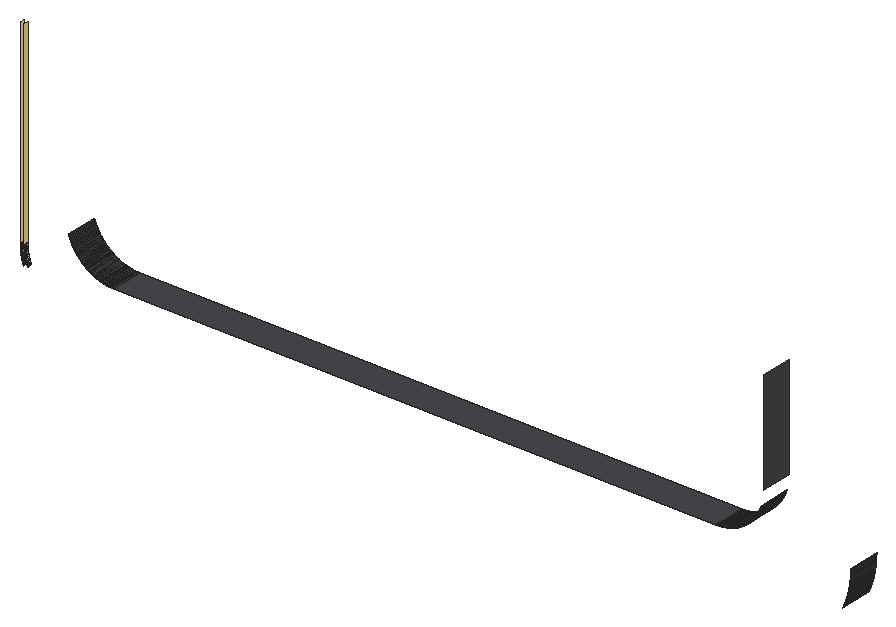
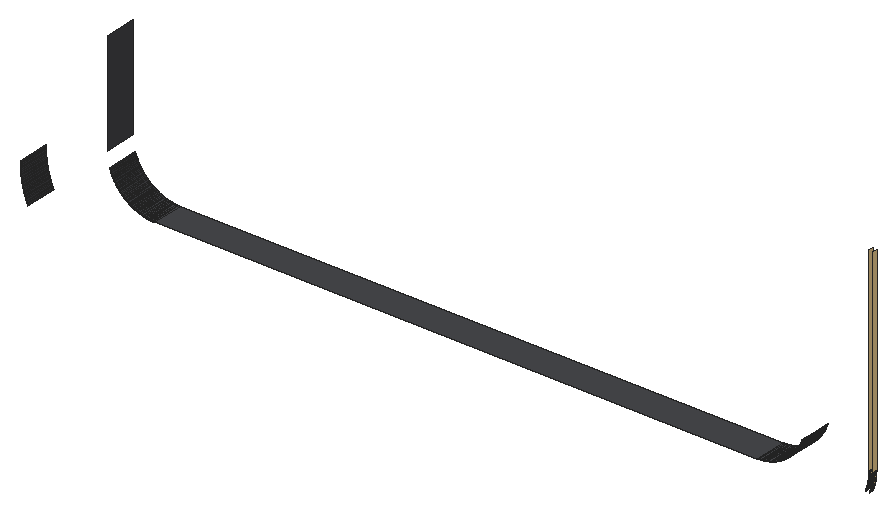
# SketchUp Ruby script. Lengths in inches.
U = 1.inch
M = Sketchup.active_model
def pt(a) = Geom::Point3d.new(a.map { |v| v * U })
def face(e, loops, mat)
  f = e.add_face(loops[0].map { |a| pt(a) })
  loops[1..].each { |l| e.add_face(l.map { |a| pt(a) }).erase! }
  f.material = f.back_material = mat if mat
  f
end
# faces: each face lists its corners as indices into pts; further lists are holes
def faces(e, pts, list, mat = nil) = list.each { |f| face(e, (f[0].is_a?(Array) ? f : [f]).map { |l| l.map { |i| pts[i] } }, mat) }
# xy, xz, yz: faces in a plane at the given z, y or x. An outline is a flat list of corners, or four numbers for a rectangle; further outlines are holes
def ring(l) = l.size == 4 ? [[l[0], l[1]], [l[2], l[1]], [l[2], l[3]], [l[0], l[3]]] : l.each_slice(2).to_a
def flat(e, list, mat, &to3) = list.each { |f| face(e, (f[0].is_a?(Array) ? f : [f]).map { |l| ring(l).map { |u, v| to3.(u, v) } }, mat) }
def xy(e, z, list, mat = nil) = flat(e, list, mat) { |x, y| [x, y, z] }
def xz(e, y, list, mat = nil) = flat(e, list, mat) { |x, z| [x, y, z] }
def yz(e, x, list, mat = nil) = flat(e, list, mat) { |y, z| [x, y, z] }
def lines(e, pts, list) = list.each { |a, b| e.add_line(pt(pts[a]), pt(pts[b])) }
# prism: a flat outline (further loops are holes) pulled along v
def prism(e, loops, v, mat = nil)
  f = face(e, loops, mat); d = Geom::Vector3d.new(v.map { |x| x * U })
  f.pushpull(f.normal.samedirection?(d) ? d.length : -d.length)
end
def box(e, o, s, mat = nil) = prism(e, [[o, [o[0] + s[0], o[1], o[2]], [o[0] + s[0], o[1] + s[1], o[2]], [o[0], o[1] + s[1], o[2]]]], [0, 0, s[2]], mat)
def at(x, y, z, deg = 0) = Geom::Transformation.translation(pt([x, y, z])) * Geom::Transformation.rotation(ORIGIN, Z_AXIS, deg.degrees)
def axes(o, x, y, z) = Geom::Transformation.new([*x, 0, *y, 0, *z, 0, *pt(o).to_a, 1])
def part(name) = M.definitions.add(name)
# library, detail: a bought-in or finely detailed component or shape, given as its bounding box
def library(name, o, s) = part(name).tap { |d| box(d.entities, o, s) }
def detail(e, o, s) = box(e.add_group.entities, o, s)
def put(e, d, t, mat = nil) = e.add_instance(d, t).tap { |i| i.material = mat if mat }
def group(e, t, mat = nil) = e.add_group.tap { |g| g.transformation = t; g.material = mat if mat }.entities
root = M.entities
M.materials.add("1432 AP 8245 TAR ROAD").color = [71, 72, 75]
M.materials.add("Outer Light").color = [251, 217, 152]
xy(root,188.79,[[293.76,95.37,294,107.37],[294,95.37,522,107.37],[522,95.37,522.2,107.37]],"1432 AP 8245 TAR ROAD")
xy(root,188.8,[[522.4,95.37,522.61,107.37]],"1432 AP 8245 TAR ROAD")
yz(root,258.5,[[95.37,191.47,96.87,191.63],[95.37,191.63,96.87,191.79],[95.37,191.79,96.87,266.79]],"Outer Light")
yz(root,258.51,[[95.37,191.15,96.87,191.31]],"Outer Light")
yz(root,258.52,[[95.37,190.83,96.87,190.99]],"Outer Light")
yz(root,260,[[95.37,191.49,96.87,191.64],[95.37,191.64,96.87,191.79],[95.37,191.79,96.87,266.79]],"Outer Light")
yz(root,260.01,[[95.37,191.05,96.87,191.2],[95.37,191.2,96.87,191.34]],"Outer Light")
yz(root,540,[[95.37,206.79,107.37,245.79]],"1432 AP 8245 TAR ROAD")
yz(root,573,[[95.37,191.23,107.37,191.51],[95.37,191.51,107.37,191.79]],"1432 AP 8245 TAR ROAD")
p = [[570.04,107.37,177.49],[570.15,107.37,177.75],[570.15,95.37,177.75],[570.04,95.37,177.49],[570.26,107.37,178.02],[570.26,95.37,178.02],
  [570.37,107.37,178.28],[570.37,95.37,178.28],[570.47,107.37,178.54],[570.47,95.37,178.54],[570.58,107.37,178.8],[570.58,95.37,178.8],
  [570.68,107.37,179.07],[570.68,95.37,179.07],[570.77,107.37,179.33],[570.77,95.37,179.33],[570.87,107.37,179.6],[570.87,95.37,179.6],
  [570.97,107.37,179.86],[570.97,95.37,179.86],[571.06,107.37,180.13],[571.06,95.37,180.13],[571.15,107.37,180.4],[571.15,95.37,180.4],
  [571.24,107.37,180.67],[571.24,95.37,180.67],[571.32,107.37,180.9375],[571.32,95.37,180.9375],[571.41,107.37,181.21],[571.41,95.37,181.21],
  [571.49,107.37,181.48],[571.49,95.37,181.48],[571.57,107.37,181.75],[571.57,95.37,181.75],[571.65,107.37,182.02],[571.65,95.37,182.02],
  [571.72,107.37,182.29],[571.72,95.37,182.29],[571.8,107.37,182.57],[571.8,95.37,182.57],[571.87,107.37,182.84],[571.87,95.37,182.84],
  [571.9375,107.37,183.11],[571.9375,95.37,183.11],[572.01,107.37,183.39],[572.01,95.37,183.39],[572.07,107.37,183.66],[572.07,95.37,183.66],
  [572.13,107.37,183.9375],[572.13,95.37,183.9375],[572.19,107.37,184.22],[572.19,95.37,184.22],[572.25,107.37,184.49],[572.25,95.37,184.49],
  [259.77,95.37,184.7],[259.82,95.37,184.55],[259.82,96.87,184.55],[259.77,96.87,184.7],[259.77,96.87,184.7],[259.82,96.87,184.55],
  [259.82,95.37,184.55],[259.77,95.37,184.7],[572.31,107.37,184.77],[572.31,95.37,184.77],[259.71,95.37,184.85],[259.71,96.87,184.85],
  [259.71,96.87,184.85],[259.71,95.37,184.85],[261.39,96.87,184.66],[261.33,96.87,184.8],[261.33,95.37,184.8],[261.39,95.37,184.66],
  [259.66,95.37,185],[259.66,96.87,185],[259.66,96.87,185],[259.66,95.37,185],[261.28,96.87,184.9375],[261.28,95.37,184.9375],
  [572.36,107.37,185.05],[572.36,95.37,185.05],[261.23,96.87,185.08],[261.23,95.37,185.08],[259.61,96.87,185.15],[259.61,95.37,185.15],
  [572.41,107.37,185.32],[572.41,95.37,185.32],[261.17,96.87,185.22],[261.17,95.37,185.22],[259.55,96.87,185.3],[259.55,95.37,185.3],
  [261.125,96.87,185.36],[261.125,95.37,185.36],[259.5,96.87,185.46],[259.5,95.37,185.46],[572.46,107.37,185.6],[572.46,95.37,185.6],
  [261.07,96.87,185.5],[261.07,95.37,185.5],[259.45,96.87,185.61],[259.45,95.37,185.61],[261.02,96.87,185.64],[261.02,95.37,185.64],
  [259.41,96.87,185.76],[259.41,95.37,185.76],[260.98,96.87,185.78],[260.98,95.37,185.78],[572.51,107.37,185.88],[572.51,95.37,185.88],
  [259.36,96.87,185.92],[259.36,95.37,185.92],[260.93,96.87,185.92],[260.93,95.37,185.92],[259.3125,96.87,186.07],[259.3125,95.37,186.07],
  [260.88,96.87,186.0625],[260.88,95.37,186.0625],[572.56,107.37,186.16],[572.56,95.37,186.16],[259.27,96.87,186.23],[259.27,95.37,186.23],
  [260.84,96.87,186.21],[260.84,95.37,186.21],[259.23,96.87,186.38],[259.23,95.37,186.38],[260.8,96.87,186.35],[260.8,95.37,186.35],
  [572.6,107.37,186.44],[572.6,95.37,186.44],[260.75,96.87,186.49],[260.75,95.37,186.49],[259.18,96.87,186.54],[259.18,95.37,186.54],
  [259.18,95.37,186.54],[259.23,95.37,186.38],[259.23,96.87,186.38],[259.18,96.87,186.54],[572.64,107.37,186.72],[572.64,95.37,186.72],
  [259.14,96.87,186.69],[259.14,95.37,186.69],[259.14,95.37,186.69],[259.14,96.87,186.69],[260.71,96.87,186.63],[260.71,95.37,186.63],
  [260.67,96.87,186.78],[260.67,95.37,186.78],[259.1,96.87,186.85],[259.1,95.37,186.85],[259.1,95.37,186.85],[259.1,96.87,186.85],
  [572.68,107.37,187],[572.68,95.37,187],[260.63,96.87,186.92],[260.63,95.37,186.92],[259.07,96.87,187.01],[259.07,95.37,187.01],
  [259.07,95.37,187.01],[259.07,96.87,187.01],[260.6,96.87,187.07],[260.6,95.37,187.07],[259.03,96.87,187.16],[259.03,95.37,187.16],
  [259.03,95.37,187.16],[259.03,96.87,187.16],[572.72,107.37,187.28],[572.72,95.37,187.28],[260.56,96.87,187.21],[260.56,95.37,187.21],
  [258.99,96.87,187.32],[258.99,95.37,187.32],[258.99,95.37,187.32],[258.99,96.87,187.32],[260.52,96.87,187.36],[260.52,95.37,187.36],
  [258.96,96.87,187.48],[258.96,95.37,187.48],[258.96,95.37,187.48],[258.96,96.87,187.48],[572.75,107.37,187.5625],[572.75,95.37,187.5625],
  [260.49,96.87,187.5],[260.49,95.37,187.5],[258.93,96.87,187.63],[258.93,95.37,187.63],[258.93,95.37,187.63],[258.93,96.87,187.63],
  [260.46,96.87,187.65],[260.46,95.37,187.65],[258.89,96.87,187.79],[258.89,95.37,187.79],[260.43,96.87,187.79],[260.43,95.37,187.79],
  [572.78,107.37,187.84],[572.78,95.37,187.84],[258.86,96.87,187.95],[258.86,95.37,187.95],[260.39,96.87,187.9375],[260.39,95.37,187.9375],
  [572.8125,107.37,188.12],[572.8125,95.37,188.12],[260.37,96.87,188.09],[260.37,95.37,188.09],[258.83,96.87,188.11],[258.83,95.37,188.11],
  [258.81,96.87,188.27],[258.81,95.37,188.27],[260.34,96.87,188.23],[260.34,95.37,188.23],[572.84,107.37,188.4],[572.84,95.37,188.4],
  [260.31,96.87,188.38],[260.31,95.37,188.38],[258.78,96.87,188.43],[258.78,95.37,188.43],[258.75,96.87,188.59],[258.75,95.37,188.59],
  [260.28,96.87,188.53],[260.28,95.37,188.53],[572.87,107.37,188.6875],[572.87,95.37,188.6875],[260.26,96.87,188.67],[260.26,95.37,188.67],
  [258.73,96.87,188.74],[258.73,95.37,188.74],[258.7,96.87,188.9],[258.7,95.37,188.9],[260.23,96.87,188.82],[260.23,95.37,188.82],
  [572.89,107.37,188.97],[572.89,95.37,188.97],[260.21,96.87,188.97],[260.21,95.37,188.97],[292.59,107.37,188.85],[292.35,107.37,188.87],
  [292.35,95.37,188.87],[292.59,95.37,188.85],[292.82,107.37,188.83],[292.82,95.37,188.83],[293.06,107.37,188.82],[293.06,95.37,188.82],
  [293.29,107.37,188.81],[293.29,95.37,188.81],[293.53,107.37,188.8],[293.53,95.37,188.8],[293.76,107.37,188.79],[293.76,95.37,188.79],
  [522.4,107.37,188.8],[522.2,107.37,188.79],[522.2,95.37,188.79],[522.4,95.37,188.8],[522.81,107.37,188.81],[522.61,107.37,188.8],
  [522.61,95.37,188.8],[522.81,95.37,188.81],[523.01,107.37,188.82],[523.01,95.37,188.82],[523.21,107.37,188.83],[523.21,95.37,188.83],
  [523.41,107.37,188.85],[523.41,95.37,188.85],[523.61,107.37,188.86],[523.61,95.37,188.86],[258.68,96.87,189.0625],[258.68,95.37,189.0625],
  [291.65,107.37,188.95],[291.42,107.37,188.98],[291.42,95.37,188.98],[291.65,95.37,188.95],[291.88,107.37,188.92],[291.88,95.37,188.92],
  [292.12,107.37,188.89],[292.12,95.37,188.89],[523.81,107.37,188.88],[523.81,95.37,188.88],[524.02,107.37,188.91],[524.02,95.37,188.91],
  [524.22,107.37,188.93],[524.22,95.37,188.93],[524.42,107.37,188.95],[524.42,95.37,188.95],[260.19,96.87,189.11],[260.19,95.37,189.11],
  [291.18,107.37,189.01],[290.95,107.37,189.05],[290.95,95.37,189.05],[291.18,95.37,189.01],[524.62,107.37,188.98],[524.62,95.37,188.98],
  [524.82,107.37,189.01],[524.82,95.37,189.01],[525.02,107.37,189.05],[525.02,95.37,189.05],[525.21,107.37,189.08],[525.21,95.37,189.08],
  [572.91,107.37,189.25],[572.91,95.37,189.25],[258.66,96.87,189.22],[258.66,95.37,189.22],[260.17,96.87,189.26],[260.17,95.37,189.26],
  [290.49,107.37,189.14],[290.26,107.37,189.19],[290.26,95.37,189.19],[290.49,95.37,189.14],[290.72,107.37,189.09],[290.72,95.37,189.09],
  [525.41,107.37,189.12],[525.41,95.37,189.12],[525.61,107.37,189.16],[525.61,95.37,189.16],[258.64,96.87,189.38],[258.64,95.37,189.38],
  [290.03,107.37,189.24],[289.8,107.37,189.29],[289.8,95.37,189.29],[290.03,95.37,189.24],[525.81,107.37,189.2],[525.81,95.37,189.2],
  [526.01,107.37,189.24],[526.01,95.37,189.24],[526.2,107.37,189.29],[526.2,95.37,189.29],[572.93,107.37,189.53],[572.93,95.37,189.53],
  [260.15,96.87,189.41],[260.15,95.37,189.41],[289.57,107.37,189.35],[289.34,107.37,189.41],[289.34,95.37,189.41],[289.57,95.37,189.35],
  [526.4,107.37,189.34],[526.4,95.37,189.34],[526.59,107.37,189.39],[526.59,95.37,189.39],[258.625,96.87,189.54],[258.625,95.37,189.54],
  [260.13,96.87,189.56],[260.13,95.37,189.56],[289.11,107.37,189.47],[289.11,95.37,189.47],[526.79,107.37,189.44],[526.79,95.37,189.44],
  [526.98,107.37,189.5],[526.98,95.37,189.5],[258.61,96.87,189.7],[258.61,95.37,189.7],[288.89,107.37,189.53],[288.66,107.37,189.6],
  [288.66,95.37,189.6],[288.89,95.37,189.53],[527.18,107.37,189.55],[527.18,95.37,189.55],[572.95,107.37,189.8125],[572.95,95.37,189.8125],
  [260.11,96.87,189.71],[260.11,95.37,189.71],[288.4375,107.37,189.67],[288.4375,95.37,189.67],[527.37,107.37,189.61],[527.37,95.37,189.61],
  [527.5625,107.37,189.67],[527.5625,95.37,189.67],[258.59,96.87,189.86],[258.59,95.37,189.86],[260.1,96.87,189.86],[260.1,95.37,189.86],
  [288.21,107.37,189.75],[287.99,107.37,189.82],[287.99,95.37,189.82],[288.21,95.37,189.75],[527.75,107.37,189.74],[527.75,95.37,189.74],
  [527.95,107.37,189.8],[527.95,95.37,189.8],[287.77,107.37,189.9],[287.77,95.37,189.9],[528.14,107.37,189.87],[528.14,95.37,189.87],
  [572.96,107.37,190.1],[572.96,95.37,190.1],[258.58,96.87,190.02],[258.58,95.37,190.02],[260.08,96.87,190],[260.08,95.37,190],
  [287.55,107.37,189.99],[287.55,95.37,189.99],[528.32,107.37,189.94],[528.32,95.37,189.94],[528.51,107.37,190.01],[528.51,95.37,190.01],
  [258.5625,96.87,190.18],[258.5625,95.37,190.18],[260.07,96.87,190.15],[260.07,95.37,190.15],[287.33,107.37,190.07],[287.33,95.37,190.07],
  [528.7,107.37,190.09],[528.7,95.37,190.09],[287.11,107.37,190.16],[287.11,95.37,190.16],[528.89,107.37,190.16],[528.89,95.37,190.16],
  [572.97,107.37,190.38],[572.97,95.37,190.38],[258.55,96.87,190.34],[258.55,95.37,190.34],[260.06,96.87,190.3],[260.06,95.37,190.3],
  [286.89,107.37,190.25],[286.89,95.37,190.25],[529.07,107.37,190.24],[529.07,95.37,190.24],[529.26,107.37,190.32],[529.26,95.37,190.32],
  [258.54,96.87,190.5],[258.54,95.37,190.5],[260.05,96.87,190.45],[260.05,95.37,190.45],[286.68,107.37,190.35],[286.46,107.37,190.45],
  [286.46,95.37,190.45],[286.68,95.37,190.35],[529.44,107.37,190.4],[529.44,95.37,190.4],[286.25,107.37,190.55],[286.25,95.37,190.55],
  [529.63,107.37,190.49],[529.63,95.37,190.49],[572.98,107.37,190.66],[572.98,95.37,190.66],[258.53,96.87,190.67],[258.53,95.37,190.67],
  [260.04,96.87,190.6],[260.04,95.37,190.6],[286.04,107.37,190.65],[286.04,95.37,190.65],[529.81,107.37,190.57],[529.81,95.37,190.57],
  [260.03,96.87,190.75],[260.03,95.37,190.75],[285.83,107.37,190.75],[285.83,95.37,190.75],[529.99,107.37,190.66],[529.99,95.37,190.66],
  [258.52,96.87,190.83],[258.52,95.37,190.83],[260.02,96.87,190.9],[260.02,95.37,190.9],[530.17,107.37,190.75],[530.17,95.37,190.75],
  [572.99,107.37,190.94],[572.99,95.37,190.94],[285.62,107.37,190.86],[285.62,95.37,190.86],[530.35,107.37,190.85],[530.35,95.37,190.85],
  [530.53,107.37,190.94],[530.53,95.37,190.94],[260.01,96.87,191.05],[260.01,95.37,191.05],[285.41,107.37,190.97],[285.41,95.37,190.97],
  [530.71,107.37,191.04],[530.71,95.37,191.04],[573,107.37,191.23],[573,95.37,191.23],[258.51,96.87,191.15],[258.52,96.87,190.99],
  [258.52,95.37,190.99],[258.51,95.37,191.15],[285.2,107.37,191.09],[285.2,95.37,191.09],[530.88,107.37,191.14],[530.88,95.37,191.14],
  [285,107.37,191.2],[285,95.37,191.2],[531.06,107.37,191.24],[531.06,95.37,191.24],[284.8,107.37,191.32],[284.8,95.37,191.32],
  [531.23,107.37,191.34],[531.23,95.37,191.34],[258.5,96.87,191.47],[258.51,96.87,191.31],[258.51,95.37,191.31],[258.5,95.37,191.47],
  [260.01,96.87,191.34],[260,96.87,191.49],[260,95.37,191.49],[260.01,95.37,191.34],[284.6,107.37,191.44],[284.6,95.37,191.44],
  [531.4,107.37,191.44],[531.4,95.37,191.44],[284.39,107.37,191.57],[284.39,95.37,191.57],[531.58,107.37,191.55],[531.58,95.37,191.55],
  [284.2,107.37,191.7],[284.2,95.37,191.7],[531.75,107.37,191.66],[531.75,95.37,191.66],[284,107.37,191.83],[284,95.37,191.83],
  [531.92,107.37,191.77],[531.92,95.37,191.77],[283.8,107.37,191.96],[283.8,95.37,191.96],[532.08,107.37,191.88],[532.08,95.37,191.88],
  [532.25,107.37,192],[532.25,95.37,192],[283.61,107.37,192.09],[283.61,95.37,192.09],[532.42,107.37,192.11],[532.42,95.37,192.11],
  [283.42,107.37,192.23],[283.42,95.37,192.23],[532.58,107.37,192.23],[532.58,95.37,192.23],[283.23,107.37,192.37],[283.23,95.37,192.37],
  [532.74,107.37,192.35],[532.74,95.37,192.35],[532.9,107.37,192.47],[532.9,95.37,192.47],[283.04,107.37,192.51],[283.04,95.37,192.51],
  [282.86,107.37,192.66],[282.86,95.37,192.66],[533.0625,107.37,192.59],[533.0625,95.37,192.59],[533.22,107.37,192.72],[533.22,95.37,192.72],
  [282.67,107.37,192.8],[282.67,95.37,192.8],[533.38,107.37,192.85],[533.38,95.37,192.85],[282.49,107.37,192.95],[282.49,95.37,192.95],
  [533.54,107.37,192.97],[533.54,95.37,192.97],[282.31,107.37,193.1],[282.31,95.37,193.1],[533.69,107.37,193.1],[533.69,95.37,193.1],
  [282.13,107.37,193.26],[282.13,95.37,193.26],[533.84,107.37,193.24],[533.84,95.37,193.24],[533.99,107.37,193.37],[533.99,95.37,193.37],
  [281.96,107.37,193.42],[281.96,95.37,193.42],[281.78,107.37,193.57],[281.78,95.37,193.57],[534.14,107.37,193.51],[534.14,95.37,193.51],
  [534.29,107.37,193.64],[534.29,95.37,193.64],[281.61,107.37,193.74],[281.61,95.37,193.74],[534.4375,107.37,193.78],[534.4375,95.37,193.78],
  [281.44,107.37,193.9],[281.44,95.37,193.9],[534.58,107.37,193.92],[534.58,95.37,193.92],[281.27,107.37,194.0625],[281.27,95.37,194.0625],
  [534.73,107.37,194.0625],[534.73,95.37,194.0625],[281.11,107.37,194.23],[281.11,95.37,194.23],[534.87,107.37,194.21],[534.87,95.37,194.21],
  [280.94,107.37,194.4],[280.94,95.37,194.4],[535.01,107.37,194.35],[535.01,95.37,194.35],[280.78,107.37,194.57],[280.78,95.37,194.57],
  [535.15,107.37,194.5],[535.15,95.37,194.5],[535.29,107.37,194.65],[535.29,95.37,194.65],[280.625,107.37,194.75],[280.625,95.37,194.75],
  [535.42,107.37,194.8],[535.42,95.37,194.8],[280.47,107.37,194.92],[280.47,95.37,194.92],[535.56,107.37,194.95],[535.56,95.37,194.95],
  [280.3125,107.37,195.1],[280.3125,95.37,195.1],[535.6875,107.37,195.1],[535.6875,95.37,195.1],[280.16,107.37,195.28],[280.16,95.37,195.28],
  [535.82,107.37,195.26],[535.82,95.37,195.26],[280.01,107.37,195.46],[280.01,95.37,195.46],[535.95,107.37,195.41],[535.95,95.37,195.41],
  [536.07,107.37,195.57],[536.07,95.37,195.57],[279.86,107.37,195.65],[279.86,95.37,195.65],[279.72,107.37,195.83],[279.72,95.37,195.83],
  [536.2,107.37,195.73],[536.2,95.37,195.73],[536.32,107.37,195.89],[536.32,95.37,195.89],[279.58,107.37,196.02],[279.58,95.37,196.02],
  [536.44,107.37,196.05],[536.44,95.37,196.05],[279.4375,107.37,196.21],[279.4375,95.37,196.21],[536.5625,107.37,196.21],[536.5625,95.37,196.21],
  [279.3,107.37,196.4],[279.3,95.37,196.4],[536.68,107.37,196.375],[536.68,95.37,196.375],[279.17,107.37,196.6],[279.17,95.37,196.6],
  [536.8,107.37,196.54],[536.8,95.37,196.54],[536.91,107.37,196.71],[536.91,95.37,196.71],[279.03,107.37,196.79],[279.03,95.37,196.79],
  [537.02,107.37,196.875],[537.02,95.37,196.875],[278.9,107.37,196.99],[278.9,95.37,196.99],[537.13,107.37,197.05],[537.13,95.37,197.05],
  [278.78,107.37,197.1875],[278.78,95.37,197.1875],[537.24,107.37,197.22],[537.24,95.37,197.22],[278.65,107.37,197.39],[278.65,95.37,197.39],
  [537.35,107.37,197.39],[537.35,95.37,197.39],[278.53,107.37,197.59],[278.53,95.37,197.59],[537.45,107.37,197.56],[537.45,95.37,197.56],
  [278.41,107.37,197.79],[278.41,95.37,197.79],[537.55,107.37,197.73],[537.55,95.37,197.73],[537.66,107.37,197.91],[537.66,95.37,197.91],
  [278.3,107.37,198],[278.3,95.37,198],[537.75,107.37,198.09],[537.75,95.37,198.09],[278.18,107.37,198.2],[278.18,95.37,198.2],
  [537.85,107.37,198.26],[537.85,95.37,198.26],[278.07,107.37,198.41],[278.07,95.37,198.41],[537.95,107.37,198.44],[537.95,95.37,198.44],
  [277.96,107.37,198.62],[277.96,95.37,198.62],[538.04,107.37,198.62],[538.04,95.37,198.62],[277.86,107.37,198.83],[277.86,95.37,198.83],
  [538.13,107.37,198.8],[538.13,95.37,198.8],[277.75,107.37,199.04],[277.75,95.37,199.04],[538.22,107.37,198.98],[538.22,95.37,198.98],
  [277.65,107.37,199.26],[277.65,95.37,199.26],[538.3,107.37,199.16],[538.3,95.37,199.16],[538.39,107.37,199.35],[538.39,95.37,199.35],
  [277.56,107.37,199.47],[277.56,95.37,199.47],[538.47,107.37,199.53],[538.47,95.37,199.53],[277.46,107.37,199.6875],[277.46,95.37,199.6875],
  [538.55,107.37,199.72],[538.55,95.37,199.72],[277.37,107.37,199.9],[277.37,95.37,199.9],[538.63,107.37,199.9],[538.63,95.37,199.9],
  [277.28,107.37,200.12],[277.28,95.37,200.12],[538.71,107.37,200.09],[538.71,95.37,200.09],[277.2,107.37,200.34],[277.2,95.37,200.34],
  [538.78,107.37,200.28],[538.78,95.37,200.28],[277.11,107.37,200.5625],[277.11,95.37,200.5625],[538.85,107.37,200.47],[538.85,95.37,200.47],
  [538.92,107.37,200.66],[538.92,95.37,200.66],[277.03,107.37,200.78],[277.03,95.37,200.78],[538.99,107.37,200.85],[538.99,95.37,200.85],
  [276.96,107.37,201.01],[276.96,95.37,201.01],[539.06,107.37,201.04],[539.06,95.37,201.04],[276.88,107.37,201.23],[276.88,95.37,201.23],
  [539.12,107.37,201.23],[539.12,95.37,201.23]]
faces(root,p,[[0,1,2,3],[1,4,5,2],[4,6,7,5],[6,8,9,7],[8,10,11,9],[10,12,13,11],[12,14,15,13],[14,16,17,15],
  [16,18,19,17],[18,20,21,19],[20,22,23,21],[22,24,25,23],[24,26,27,25],[26,28,29,27],[28,30,31,29],[30,32,33,31],
  [32,34,35,33],[34,36,37,35],[36,38,39,37],[38,40,41,39],[40,42,43,41],[42,44,45,43],[44,46,47,45],[46,48,49,47],
  [48,50,51,49],[50,52,53,51],[54,55,56,57],[52,62,63,53],[64,54,57,65],[72,64,65,73],[62,78,79,63],[78,84,85,79],
  [84,94,95,85],[94,106,107,95],[106,116,117,107],[116,126,127,117],[132,133,134,135],[126,136,137,127],[140,132,135,141],[148,140,141,149],
  [136,150,151,137],[156,148,149,157],[162,156,157,163],[150,164,165,151],[170,162,163,171],[176,170,171,177],[164,178,179,165],[184,176,177,185],
  [178,192,193,179],[192,198,199,193],[198,208,209,199],[208,218,219,209],[218,228,229,219],[232,233,234,235],[236,232,235,237],[238,236,237,239],
  [240,238,239,241],[242,240,241,243],[244,242,243,245],[246,247,248,249],[250,251,252,253],[254,250,253,255],[256,254,255,257],[258,256,257,259],
  [260,258,259,261],[264,265,266,267],[268,264,267,269],[270,268,269,271],[233,270,271,234],[272,260,261,273],[274,272,273,275],[276,274,275,277],
  [278,276,277,279],[282,283,284,285],[265,282,285,266],[286,278,279,287],[288,286,287,289],[290,288,289,291],[292,290,291,293],[228,294,295,229],
  [300,301,302,303],[304,300,303,305],[283,304,305,284],[306,292,293,307],[308,306,307,309],[312,313,314,315],[301,312,315,302],[316,308,309,317],
  [318,316,317,319],[320,318,319,321],[294,322,323,295],[326,327,328,329],[313,326,329,314],[330,320,321,331],[332,330,331,333],[327,338,339,328],
  [340,332,333,341],[342,340,341,343],[346,347,348,349],[338,346,349,339],[350,342,343,351],[322,352,353,323],[347,356,357,348],[358,350,351,359],
  [360,358,359,361],[366,367,368,369],[356,366,369,357],[370,360,361,371],[372,370,371,373],[367,374,375,368],[376,372,373,377],[352,378,379,353],
  [374,384,385,375],[386,376,377,387],[388,386,387,389],[384,394,395,385],[396,388,389,397],[394,398,399,395],[400,396,397,401],[378,402,403,379],
  [398,408,409,399],[410,400,401,411],[412,410,411,413],[418,419,420,421],[408,418,421,409],[422,412,413,423],[419,424,425,420],[426,422,423,427],
  [402,428,429,403],[424,434,435,425],[436,426,427,437],[434,440,441,435],[442,436,437,443],[448,442,443,449],[428,450,451,429],[440,452,453,441],
  [454,448,449,455],[456,454,455,457],[452,460,461,453],[462,456,457,463],[450,464,465,451],[460,470,471,461],[472,462,463,473],[470,474,475,471],
  [476,472,473,477],[474,478,479,475],[480,476,477,481],[478,490,491,479],[492,480,481,493],[490,494,495,491],[496,492,493,497],[494,498,499,495],
  [500,496,497,501],[498,502,503,499],[504,500,501,505],[502,506,507,503],[508,504,505,509],[510,508,509,511],[506,512,513,507],[514,510,511,515],
  [512,516,517,513],[518,514,515,519],[516,520,521,517],[522,518,519,523],[524,522,523,525],[520,526,527,521],[526,528,529,527],[530,524,525,531],
  [532,530,531,533],[528,534,535,529],[536,532,533,537],[534,538,539,535],[540,536,537,541],[538,542,543,539],[544,540,541,545],[542,546,547,543],
  [548,544,545,549],[550,548,549,551],[546,552,553,547],[552,554,555,553],[556,550,551,557],[558,556,557,559],[554,560,561,555],[562,558,559,563],
  [560,564,565,561],[566,562,563,567],[564,568,569,565],[570,566,567,571],[568,572,573,569],[574,570,571,575],[572,576,577,573],[578,574,575,579],
  [576,580,581,577],[582,578,579,583],[584,582,583,585],[580,586,587,581],[588,584,585,589],[586,590,591,587],[592,588,589,593],[590,594,595,591],
  [596,592,593,597],[594,598,599,595],[600,596,597,601],[598,602,603,599],[604,600,601,605],[606,604,605,607],[602,608,609,603],[608,610,611,609],
  [612,606,607,613],[614,612,613,615],[610,616,617,611],[618,614,615,619],[616,620,621,617],[622,618,619,623],[620,624,625,621],[626,622,623,627],
  [624,628,629,625],[630,626,627,631],[632,630,631,633],[628,634,635,629],[636,632,633,637],[634,638,639,635],[640,636,637,641],[638,642,643,639],
  [644,640,641,645],[642,646,647,643],[648,644,645,649],[646,650,651,647],[652,648,649,653],[650,654,655,651],[656,652,653,657],[658,656,657,659],
  [654,660,661,655],[662,658,659,663],[660,664,665,661],[666,662,663,667],[664,668,669,665],[670,666,667,671],[668,672,673,669],[674,670,671,675],
  [672,676,677,673],[678,674,675,679],[676,680,681,677],[682,678,679,683],[680,684,685,681],[686,682,683,687],[688,686,687,689],[684,690,691,685],
  [692,688,689,693],[690,694,695,691],[696,692,693,697],[694,698,699,695],[700,696,697,701],[698,702,703,699],[704,700,701,705],[702,706,707,703],
  [708,704,705,709],[706,710,711,707],[712,708,709,713],[714,712,713,715],[710,716,717,711],[718,714,715,719],[716,720,721,717],[722,718,719,723],
  [720,724,725,721],[726,722,723,727]],"1432 AP 8245 TAR ROAD")
faces(root,p,[[58,59,60,61],[66,58,61,67],[68,69,70,71],[74,66,67,75],[69,76,77,70],[76,80,81,77],[82,74,75,83],[80,86,87,81],
  [88,82,83,89],[86,90,91,87],[92,88,89,93],[90,96,97,91],[98,92,93,99],[96,100,101,97],[102,98,99,103],[100,104,105,101],
  [108,102,103,109],[104,110,111,105],[112,108,109,113],[110,114,115,111],[118,112,113,119],[114,120,121,115],[122,118,119,123],[120,124,125,121],
  [124,128,129,125],[130,122,123,131],[138,130,131,139],[128,142,143,129],[142,144,145,143],[146,138,139,147],[144,152,153,145],[154,146,147,155],
  [152,158,159,153],[160,154,155,161],[158,166,167,159],[168,160,161,169],[166,172,173,167],[174,168,169,175],[172,180,181,173],[182,174,175,183],
  [180,186,187,181],[188,182,183,189],[186,190,191,187],[194,188,189,195],[190,196,197,191],[196,200,201,197],[202,194,195,203],[204,202,203,205],
  [200,206,207,201],[206,210,211,207],[212,204,205,213],[214,212,213,215],[210,216,217,211],[216,220,221,217],[222,214,215,223],[224,222,223,225],
  [220,226,227,221],[226,230,231,227],[262,224,225,263],[230,280,281,231],[296,262,263,297],[280,298,299,281],[310,296,297,311],[298,324,325,299],
  [334,310,311,335],[324,336,337,325],[344,334,335,345],[336,354,355,337],[362,344,345,363],[354,364,365,355],[380,362,363,381],[364,382,383,365],
  [390,380,381,391],[382,392,393,383],[404,390,391,405],[392,406,407,393],[414,404,405,415],[406,416,417,407],[430,414,415,431],[416,432,433,417],
  [432,438,439,433],[444,430,431,445],[438,446,447,439],[446,458,459,447],[466,467,468,469],[482,483,484,485],[486,487,488,489]],"Outer Light")
